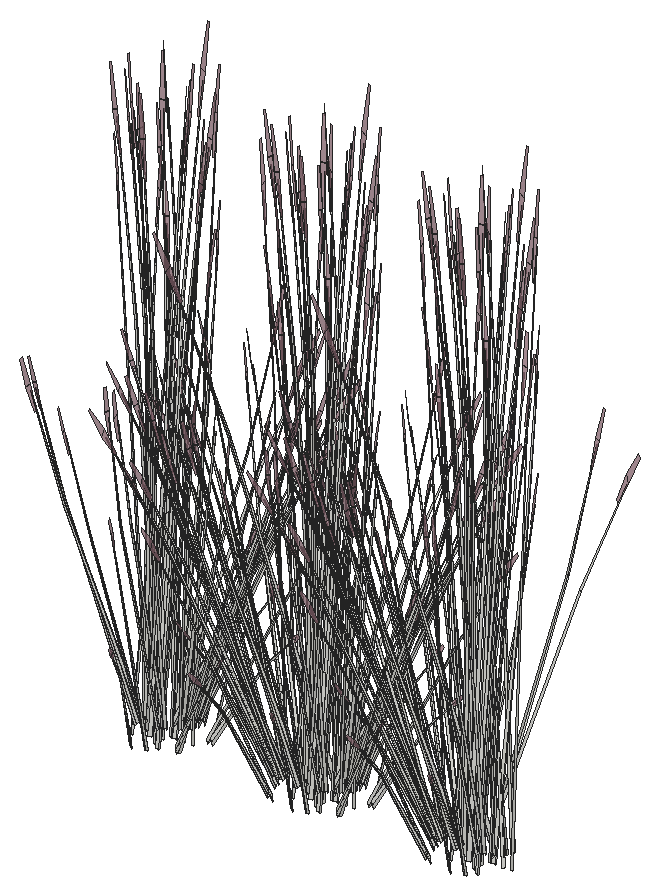
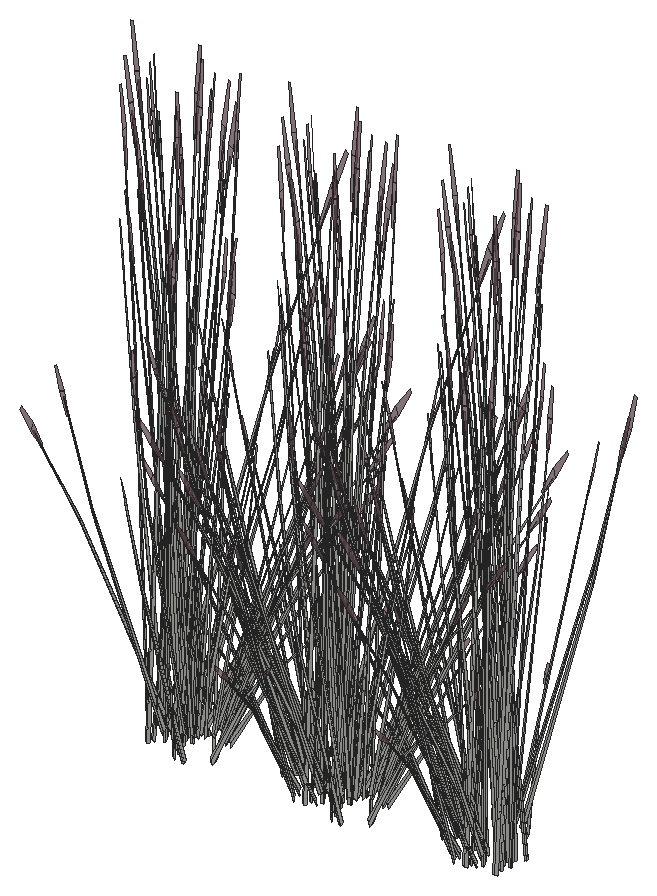
# SketchUp Ruby script. Lengths in inches.
U = 1.inch
M = Sketchup.active_model
def pt(a) = Geom::Point3d.new(a.map { |v| v * U })
def face(e, loops, mat)
  f = e.add_face(loops[0].map { |a| pt(a) })
  loops[1..].each { |l| e.add_face(l.map { |a| pt(a) }).erase! }
  f.material = f.back_material = mat if mat
  f
end
# faces: each face lists its corners as indices into pts; further lists are holes
def faces(e, pts, list, mat = nil) = list.each { |f| face(e, (f[0].is_a?(Array) ? f : [f]).map { |l| l.map { |i| pts[i] } }, mat) }
# xy, xz, yz: faces in a plane at the given z, y or x. An outline is a flat list of corners, or four numbers for a rectangle; further outlines are holes
def ring(l) = l.size == 4 ? [[l[0], l[1]], [l[2], l[1]], [l[2], l[3]], [l[0], l[3]]] : l.each_slice(2).to_a
def flat(e, list, mat, &to3) = list.each { |f| face(e, (f[0].is_a?(Array) ? f : [f]).map { |l| ring(l).map { |u, v| to3.(u, v) } }, mat) }
def xy(e, z, list, mat = nil) = flat(e, list, mat) { |x, y| [x, y, z] }
def xz(e, y, list, mat = nil) = flat(e, list, mat) { |x, z| [x, y, z] }
def yz(e, x, list, mat = nil) = flat(e, list, mat) { |y, z| [x, y, z] }
def lines(e, pts, list) = list.each { |a, b| e.add_line(pt(pts[a]), pt(pts[b])) }
# prism: a flat outline (further loops are holes) pulled along v
def prism(e, loops, v, mat = nil)
  f = face(e, loops, mat); d = Geom::Vector3d.new(v.map { |x| x * U })
  f.pushpull(f.normal.samedirection?(d) ? d.length : -d.length)
end
def box(e, o, s, mat = nil) = prism(e, [[o, [o[0] + s[0], o[1], o[2]], [o[0] + s[0], o[1] + s[1], o[2]], [o[0], o[1] + s[1], o[2]]]], [0, 0, s[2]], mat)
def at(x, y, z, deg = 0) = Geom::Transformation.translation(pt([x, y, z])) * Geom::Transformation.rotation(ORIGIN, Z_AXIS, deg.degrees)
def axes(o, x, y, z) = Geom::Transformation.new([*x, 0, *y, 0, *z, 0, *pt(o).to_a, 1])
def part(name) = M.definitions.add(name)
# library, detail: a bought-in or finely detailed component or shape, given as its bounding box
def library(name, o, s) = part(name).tap { |d| box(d.entities, o, s) }
def detail(e, o, s) = box(e.add_group.entities, o, s)
def put(e, d, t, mat = nil) = e.add_instance(d, t).tap { |i| i.material = mat if mat }
def group(e, t, mat = nil) = e.add_group.tap { |g| g.transformation = t; g.material = mat if mat }.entities
root = M.entities
M.materials.add("LightPink_Translucent").color = [144, 107, 117]
M.materials["LightPink_Translucent"].alpha = 0.75
c1 = part("blade")
p = [[2.15,0.21,22],[0,0.17,0],[0.09,0.45,0],[2.18,0.31,22],[2.29,0.31,22],[0.38,0.45,0],
  [2.48,0.24,33],[2.49,0.24,33],[2.48,0.22,33]]
faces(c1.entities,p,[[0,1,2,3],[4,5,2,3],[6,3,4,7],[8,0,3,6]])
c2 = part("seeds")
p = [[0.3,-0.1,1.38],[-0.01,-0.03,1.59],[-0.01,-0.03,0.03],[0.14,-0.07,-0.07],[0.29,-0.03,3],[0.15,0.01,3.11]]
faces(c2.entities,p,[[0,1,2,3],[1,0,4,5]],"LightPink_Translucent")
c3 = part("blade with seeds")
put(c3.entities,c1,at(0,0,0))
put(c3.entities,c2,axes([2.4,0.25,30.99],[1.5799,-0.05474,1.17369],[-0.12525,1.92788,0.29478],[-0.07173,-0.02425,1.56792]))
put(root,c3,axes([278.78,51.1875,259.68],[-0.7469,-0.15318,-0.51099],[0.25601,-0.52518,-0.3958],[-0.06849,-0.21144,0.97773]))
put(root,c3,axes([278.08,54.07,257.36],[0.96033,0.12874,0.45755],[-0.19544,0.7271,0.17955],[-0.14034,-0.07021,1.58856]))
put(root,c3,axes([277.83,53.94,257.72],[-0.36864,0.55059,0.44739],[-0.76598,-0.26498,-0.21531],[0,-0.12692,1.43643]))
put(root,c3,axes([279.05,51.29,259.98],[-0.36264,-0.49684,-0.71045],[0.74649,-0.27689,0.08574],[-0.0848,-0.24006,1.00501]))
put(root,c3,axes([277.57,55.23,257.47],[0.81646,-0.16218,0.17642],[0.20161,0.60355,0.35086],[-0.07282,-0.08794,1.60407]))
put(root,c3,axes([280,55.27,257.47],[0.21949,-0.60727,0.17642],[0.8032,0.17185,0.35086],[-0.13875,0.00296,1.60407]))
put(root,c3,axes([279.625,54.46,257.62],[0.56134,0.36712,0.1448],[-0.46823,0.41419,-0.41347],[-0.13033,0.05599,1.26744]))
put(root,c3,axes([279.61,54.19,257.72],[0.82508,-0.03772,0.44739],[0.07462,0.62614,-0.21531],[-0.14771,0.06346,1.43643]))
put(root,c3,axes([280.22,55.59,257.48],[0.7111,-0.30552,0.49651],[0.42504,0.54784,0],[-0.16196,0.06958,1.57504]))
put(root,c3,axes([279.12,50.87,259.53],[0.22906,-0.4699,-0.35414],[0.66828,0.13705,0.4572],[-0.06128,-0.18919,0.87481]))
put(root,c3,axes([278,53.4,257.36],[0.33034,0.68327,0.45755],[-0.94388,0.2376,0.17955],[0.01154,-0.12555,1.58856]))
put(root,c3,axes([281.25,53.72,257.47],[-0.59697,-0.44509,0.17642],[0.60159,-0.4317,0.35086],[-0.06593,0.0909,1.60407]))
put(root,c3,axes([278.3,53.59,257.43],[0.8561,0.29616,0.24065],[-0.41201,0.61537,0.50002],[0,-0.14185,1.60543]))
put(root,c3,axes([278.03,53.18,257.72],[-0.82508,0.03772,0.44739],[-0.07462,-0.62614,-0.21531],[0.14771,-0.06346,1.43643]))
put(root,c3,axes([277.64,52.1,257.47],[-0.21949,0.60727,0.17642],[-0.8032,-0.17185,0.35086],[0.13875,-0.00296,1.60407]))
put(root,c3,axes([280.07,52.14,257.47],[-0.81646,0.16218,0.17642],[-0.20161,-0.60355,0.35086],[0.07282,0.08794,1.60407]))
put(root,c3,axes([279.24,49.875,257.77],[0.09747,0.35631,1.1486],[-0.54071,-0.19735,0.84392],[0.05818,-0.18244,0.25299]))
put(root,c3,axes([278.74,53.02,257.36],[-0.62999,0.55453,0.45755],[-0.74845,-0.4895,0.17955],[0.15188,-0.05534,1.58856]))
put(root,c3,axes([279.81,53.43,257.72],[0.36864,-0.55059,0.44739],[0.76598,0.26498,-0.21531],[0,0.12692,1.43643]))
put(root,c3,axes([278.39,56.07,259.68],[0.7469,0.15318,-0.51099],[-0.25601,0.52518,-0.3958],[0.06849,0.21144,0.97773]))
put(root,c3,axes([279.56,53.3,257.38],[-0.96033,-0.12874,0.49198],[0.19544,-0.7271,0.19306],[0.14034,0.07021,1.70813]))
put(root,c3,axes([279.01,52.92,257.72],[-0.45644,-0.51287,0.44739],[0.69137,-0.36116,-0.21531],[0.14771,0.06346,1.43643]))
put(root,c3,axes([280.125,53.55,257.62],[0.70791,-0.1782,0.1448],[0.24791,0.50885,-0.41347],[0,0.11199,1.26744]))
put(root,c3,axes([280.39,51.59,259.68],[-0.54391,-0.41056,-0.51099],[0.57458,-0.35956,-0.3958],[0.08276,-0.2086,0.97773]))
put(root,c3,axes([280.03,50.86,257.59],[-0.21597,0.12368,1.43002],[-0.64681,-0.21647,-0.30754],[0.1199,-0.26922,0.61141]))
put(root,c3,axes([281.74,53.74,257.48],[0,-0.61104,0.49651],[0.85008,0,0],[0,0.13917,1.57504]))
put(root,c3,axes([278.82,54.98,258.875],[-0.17368,-0.19618,1.71376],[0.80256,-0.16516,0.13857],[0.18139,0.30799,0.73262]))
put(root,c3,axes([279.32,52.78,257.62],[0.14658,-0.54532,0.1448],[0.71613,0.09466,-0.41347],[0.13033,0.05599,1.26744]))
put(root,c3,axes([280.34,51.83,257.48],[-0.7111,-0.30552,0.49651],[0.42504,-0.54784,0],[0.16196,0.06958,1.57504]))
put(root,c3,axes([280.56,51.77,259.98],[0.01977,-0.56521,-0.71045],[0.83252,0.03796,0.08574],[0.08786,-0.23945,1.00501]))
put(root,c3,axes([280.9,51.43,259.53],[0.5141,-0.32171,-0.35414],[0.48666,0.36734,0.4572],[0.07405,-0.18664,0.87481]))
put(root,c3,axes([290.88,52.72,258.875],[0.31515,-0.01384,1.71376],[-0.20907,0.5998,0.13857],[-0.44912,-0.0371,0.73262]))
put(root,c3,axes([281.03,55.57,257.77],[-0.4278,-0.1757,1.1486],[0.5524,-0.17852,0.84392],[0.14899,0.15122,0.25299]))
put(root,c3,axes([279.5,55.38,257.59],[0.01341,-0.20255,1.43002],[0.64074,-0.22625,-0.30754],[0.1978,0.24243,0.61141]))
put(root,c3,axes([281.09,56.37,257.67],[-0.48723,-0.01916,1.0506],[0.32177,-0.40701,0.58006],[0.19248,0.1446,0.8241]))
put(root,c3,axes([291.01,53.77,258.875],[0.26363,-0.12925,1.71376],[0.22195,0.59723,0.13857],[-0.41388,0.13498,0.73262]))
put(root,c3,axes([290.19,54.79,257.59],[0.26405,0.05016,1.43002],[0.17019,0.51235,-0.30754],[-0.35868,0.0959,0.61141]))
put(root,c3,axes([279.62,51.49,258.875],[-0.14147,0.21002,1.71376],[-0.59349,-0.43464,0.13857],[0.26773,-0.27089,0.73262]))
put(root,c3,axes([292.53,53.15,258.34],[0.21597,-0.08839,1.77064],[0.07448,0.61717,0.13857],[-0.4678,0.08189,0.63284]))
put(root,c3,axes([280.06,55.8125,259.68],[0.74975,-0.14525,-0.51099],[0.13115,0.55007,-0.3958],[0.20138,0.15763,0.97773]))
put(root,c3,axes([291.82,52.16,259.98],[-0.75952,-0.01471,-0.71045],[0.05101,-0.61953,0.08574],[-0.32177,-0.06538,1.00501]))
put(root,c3,axes([291.21,52.31,257.59],[0.14835,0.17012,1.43002],[-0.34183,0.46242,-0.30754],[-0.351,-0.11053,0.61141]))
put(root,c3,axes([290.6,53.23,259.53],[-0.63144,-0.17046,-0.35414],[0.18417,-0.49731,0.4572],[-0.25423,0.0456,0.87481]))
put(root,c3,axes([291.48,51.75,258.875],[0.28223,0.10528,1.71376],[-0.58406,0.44165,0.13857],[-0.36402,-0.19924,0.73262]))
put(root,c3,axes([281.52,52.53,259.68],[-0.19519,-0.55794,-0.51099],[0.73919,-0.0976,-0.3958],[0.21183,-0.14986,0.97773]))
put(root,c3,axes([282.82,55.41,258.93],[-0.14542,-0.51365,-0.03492],[0.68734,-0.11809,-0.15832],[0.14353,0.03256,0.52218]))
put(root,c3,axes([291.04,53.49,259.68],[-0.20584,0.55581,-0.51099],[-0.70573,-0.19051,-0.3958],[-0.28414,0.05097,0.97773]))
put(root,c3,axes([291.57,52.28,259.68],[-0.55171,0.40476,-0.51099],[-0.48318,-0.42758,-0.3958],[-0.28031,-0.06159,0.97773]))
put(root,c3,axes([282.43,51.42,257.77],[-0.25308,0.31105,1.1486],[-0.21753,-0.4179,0.84392],[0.20902,-0.10472,0.25299]))
put(root,c3,axes([289.64,55.86,257.77],[0.31665,-0.27694,1.1486],[0.12495,0.43841,0.84392],[-0.22883,0.0785,0.25299]))
put(root,c3,axes([279.98,54.37,258.875],[-0.28223,-0.10528,1.71376],[0.58406,-0.44165,0.13857],[0.36402,0.19924,0.73262]))
put(root,c3,axes([291.37,51.9,259.53],[-0.43232,-0.38257,-0.35414],[0.49364,-0.36215,0.4572],[-0.25081,-0.0551,0.87481]))
put(root,c3,axes([291.98,54.17,258.875],[0.18977,-0.18775,1.71376],[0.47917,0.50677,0.13857],[-0.32866,0.23079,0.73262]))
put(root,c3,axes([290.83,54.67,259.53],[-0.66138,0.08733,-0.35414],[-0.17464,-0.49921,0.4572],[-0.18953,0.13408,0.87481]))
put(root,c3,axes([282.07,52.59,259.53],[0.66138,-0.08733,-0.35414],[0.17464,0.49921,0.4572],[0.18953,-0.13408,0.87481]))
put(root,c3,axes([281.54,52.76,259.98],[0.39688,-0.48213,-0.71045],[0.69548,0.34264,0.08574],[0.23697,-0.17468,1.00501]))
put(root,c3,axes([281.53,55.35,259.53],[0.43232,0.38257,-0.35414],[-0.49364,0.36215,0.4572],[0.25081,0.0551,0.87481]))
put(root,c3,axes([290.33,52.82,257.77],[0.48508,-0.04372,1.1486],[-0.3077,0.38525,0.84392],[-0.23971,-0.05779,0.25299]))
put(root,c3,axes([291.83,54.64,258.875],[0.14147,-0.21002,1.71376],[0.59349,0.43464,0.13857],[-0.26773,0.27089,0.73262]))
put(root,c3,axes([281.86,53.77,259.68],[0.20584,-0.55581,-0.51099],[0.70573,0.19051,-0.3958],[0.28414,-0.05097,0.97773]))
put(root,c3,axes([283.64,54.125,257.77],[-0.46945,0.10088,1.1486],[0.22097,-0.4169,0.84392],[0.24904,0.02853,0.25299]))
put(root,c3,axes([291.38,54.72,259.68],[0.19519,0.55794,-0.51099],[-0.73919,0.0976,-0.3958],[-0.21183,0.14986,0.97773]))
put(root,c3,axes([282.12,52.3125,257.59],[-0.27143,-0.0181,1.43002],[-0.27808,-0.48551,-0.30754],[0.33346,-0.13735,0.61141]))
put(root,c3,axes([282.3,54.02,259.53],[0.63144,0.17046,-0.35414],[-0.18417,0.49731,0.4572],[0.25423,-0.0456,0.87481]))
put(root,c3,axes([281.08,55.1,259.98],[0.75952,0.01471,-0.71045],[-0.05101,0.61953,0.08574],[0.32177,0.06538,1.00501]))
put(root,c3,axes([293.14,51.43,259.98],[-0.64788,-0.29534,-0.71045],[0.46044,-0.51755,0.08574],[-0.23473,-0.17635,1.00501]))
put(root,c3,axes([292.84,51.44,259.68],[-0.74975,0.14525,-0.51099],[-0.13115,-0.55007,-0.3958],[-0.20138,-0.15763,0.97773]))
put(root,c3,axes([280.58,53.41,258.875],[-0.31515,0.01384,1.71376],[0.20907,-0.5998,0.13857],[0.44912,0.0371,0.73262]))
put(root,c3,axes([281.73,53.97,259.98],[0.66765,-0.26986,-0.71045],[0.37208,0.55551,0.08574],[0.32259,-0.0631,1.00501]))
put(root,c3,axes([282.76,54.79,257.59],[-0.18299,-0.15028,1.43002],[0.23809,-0.49714,-0.30754],[0.37023,0.06735,0.61141]))
put(root,c3,axes([292.42,50.625,257.59],[-0.04601,0.19989,1.43002],[-0.67263,0.16733,-0.30754],[-0.15723,-0.25836,0.61141]))
put(root,c3,axes([292.64,51.14,258.875],[0.17368,0.19618,1.71376],[-0.80256,0.16516,0.13857],[-0.18139,-0.30799,0.73262]))
put(root,c3,axes([292.92,51.04,259.53],[-0.11735,-0.49217,-0.35414],[0.67083,-0.12996,0.4572],[-0.18018,-0.14104,0.87481]))
put(root,c3,axes([292,55.82,259.53],[-0.5141,0.32171,-0.35414],[-0.48666,-0.36734,0.4572],[-0.07405,0.18664,0.87481]))
put(root,c3,axes([294.69,54.77,258.33],[0.65659,0.2464,1.51261],[-0.64324,0.53082,0.59816],[-0.28812,-0.31461,1.26806]))
put(root,c3,axes([292.1875,50.3,257.77],[0.39634,0.21267,1.1486],[-0.57721,0.12784,0.84392],[-0.1235,-0.16344,0.25299]))
put(root,c3,axes([292.33,57.07,257.77],[-0.01966,-0.36332,1.1486],[0.49135,0.25914,0.84392],[-0.09663,0.17317,0.25299]))
put(root,c3,axes([293.03,55.54,257.48],[0.7111,0.30552,0.49651],[-0.42504,0.54784,0],[-0.16196,-0.06958,1.57504]))
put(root,c3,axes([294.05,54.59,257.62],[-0.14658,0.54532,0.1448],[-0.71613,-0.09466,-0.41347],[-0.13033,-0.05599,1.26744]))
put(root,c3,axes([291.625,53.63,257.48],[0,0.61104,0.49651],[-0.85008,0,0],[0,-0.13917,1.57504]))
put(root,c3,axes([292.51,55.67,260],[0.54391,0.41056,-0.5672],[-0.57458,0.35956,-0.43934],[-0.08276,0.2086,1.08528]))
put(root,c3,axes([295.71,53.59,257.84],[-0.02076,-0.57531,1.41272],[0.93937,0.14913,0.59816],[-0.22217,0.31481,1.3335]))
put(root,c3,axes([291.92,56.29,257.82],[0.69024,-0.1082,0.06507],[0.15868,0.43593,-0.86304],[-0.04376,0.22067,0.7736]))
put(root,c3,axes([294.51,51.1875,259.68],[-0.7469,-0.15318,-0.51099],[0.25601,-0.52518,-0.3958],[-0.06849,-0.21144,0.97773]))
put(root,c3,axes([293.81,54.07,257.36],[0.96033,0.12874,0.45755],[-0.19544,0.7271,0.17955],[-0.14034,-0.07021,1.58856]))
put(root,c3,axes([293.5625,53.94,257.72],[-0.36864,0.55059,0.44739],[-0.76598,-0.26498,-0.21531],[0,-0.12692,1.43643]))
put(root,c3,axes([294.78,51.29,259.98],[-0.36264,-0.49684,-0.71045],[0.74649,-0.27689,0.08574],[-0.0848,-0.24006,1.00501]))
put(root,c3,axes([293.29,55.23,257.47],[0.81646,-0.16218,0.17642],[0.20161,0.60355,0.35086],[-0.07282,-0.08794,1.60407]))
put(root,c3,axes([295.72,55.27,257.47],[0.21949,-0.60727,0.17642],[0.8032,0.17185,0.35086],[-0.13875,0.00296,1.60407]))
put(root,c3,axes([295.35,54.46,257.62],[0.56134,0.36712,0.1448],[-0.46823,0.41419,-0.41347],[-0.13033,0.05599,1.26744]))
put(root,c3,axes([295.34,54.19,257.72],[0.82508,-0.03772,0.44739],[0.07462,0.62614,-0.21531],[-0.14771,0.06346,1.43643]))
put(root,c3,axes([295.95,55.59,257.48],[0.7111,-0.30552,0.49651],[0.42504,0.54784,0],[-0.16196,0.06958,1.57504]))
put(root,c3,axes([294.85,50.87,259.53],[0.22906,-0.4699,-0.35414],[0.66828,0.13705,0.4572],[-0.06128,-0.18919,0.87481]))
put(root,c3,axes([293.73,53.4,257.36],[0.33034,0.68327,0.45755],[-0.94388,0.2376,0.17955],[0.01154,-0.12555,1.58856]))
put(root,c3,axes([296.98,53.72,257.47],[-0.59697,-0.44509,0.17642],[0.60159,-0.4317,0.35086],[-0.06593,0.0909,1.60407]))
put(root,c3,axes([294.03,53.59,257.43],[0.8561,0.29616,0.24065],[-0.41201,0.61537,0.50002],[0,-0.14185,1.60543]))
put(root,c3,axes([293.76,53.18,257.72],[-0.82508,0.03772,0.44739],[-0.07462,-0.62614,-0.21531],[0.14771,-0.06346,1.43643]))
put(root,c3,axes([293.37,52.1,257.47],[-0.21949,0.60727,0.17642],[-0.8032,-0.17185,0.35086],[0.13875,-0.00296,1.60407]))
put(root,c3,axes([295.8,52.14,257.47],[-0.81646,0.16218,0.17642],[-0.20161,-0.60355,0.35086],[0.07282,0.08794,1.60407]))
put(root,c3,axes([294.97,49.875,257.77],[0.09747,0.35631,1.1486],[-0.54071,-0.19735,0.84392],[0.05818,-0.18244,0.25299]))
put(root,c3,axes([294.46,53.02,257.36],[-0.62999,0.55453,0.45755],[-0.74845,-0.4895,0.17955],[0.15188,-0.05534,1.58856]))
put(root,c3,axes([295.53,53.43,257.72],[0.36864,-0.55059,0.44739],[0.76598,0.26498,-0.21531],[0,0.12692,1.43643]))
put(root,c3,axes([294.12,56.07,259.68],[0.7469,0.15318,-0.51099],[-0.25601,0.52518,-0.3958],[0.06849,0.21144,0.97773]))
put(root,c3,axes([295.29,53.3,257.38],[-0.96033,-0.12874,0.49198],[0.19544,-0.7271,0.19306],[0.14034,0.07021,1.70813]))
put(root,c3,axes([294.74,52.92,257.72],[-0.45644,-0.51287,0.44739],[0.69137,-0.36116,-0.21531],[0.14771,0.06346,1.43643]))
put(root,c3,axes([295.85,53.55,257.62],[0.70791,-0.1782,0.1448],[0.24791,0.50885,-0.41347],[0,0.11199,1.26744]))
put(root,c3,axes([296.12,51.59,259.68],[-0.54391,-0.41056,-0.51099],[0.57458,-0.35956,-0.3958],[0.08276,-0.2086,0.97773]))
put(root,c3,axes([295.76,50.86,257.59],[-0.21597,0.12368,1.43002],[-0.64681,-0.21647,-0.30754],[0.1199,-0.26922,0.61141]))
put(root,c3,axes([297.47,53.74,257.48],[0,-0.61104,0.49651],[0.85008,0,0],[0,0.13917,1.57504]))
put(root,c3,axes([294.55,54.98,258.875],[-0.17368,-0.19618,1.71376],[0.80256,-0.16516,0.13857],[0.18139,0.30799,0.73262]))
put(root,c3,axes([295.05,52.78,257.62],[0.14658,-0.54532,0.1448],[0.71613,0.09466,-0.41347],[0.13033,0.05599,1.26744]))
put(root,c3,axes([296.07,51.83,257.48],[-0.7111,-0.30552,0.49651],[0.42504,-0.54784,0],[0.16196,0.06958,1.57504]))
put(root,c3,axes([296.29,51.77,259.98],[0.01977,-0.56521,-0.71045],[0.83252,0.03796,0.08574],[0.08786,-0.23945,1.00501]))
put(root,c3,axes([306.33,52.72,258.875],[0.31515,-0.01384,1.71376],[-0.20907,0.5998,0.13857],[-0.44912,-0.0371,0.73262]))
put(root,c3,axes([296.63,51.43,259.53],[0.5141,-0.32171,-0.35414],[0.48666,0.36734,0.4572],[0.07405,-0.18664,0.87481]))
put(root,c3,axes([296.75,55.57,257.77],[-0.4278,-0.1757,1.1486],[0.5524,-0.17852,0.84392],[0.14899,0.15122,0.25299]))
put(root,c3,axes([295.23,55.38,257.59],[0.01341,-0.20255,1.43002],[0.64074,-0.22625,-0.30754],[0.1978,0.24243,0.61141]))
put(root,c3,axes([306.46,53.77,258.875],[0.26363,-0.12925,1.71376],[0.22195,0.59723,0.13857],[-0.41388,0.13498,0.73262]))
put(root,c3,axes([305.64,54.79,257.59],[0.26405,0.05016,1.43002],[0.17019,0.51235,-0.30754],[-0.35868,0.0959,0.61141]))
put(root,c3,axes([296.82,56.37,257.67],[-0.48723,-0.01916,1.0506],[0.32177,-0.40701,0.58006],[0.19248,0.1446,0.8241]))
put(root,c3,axes([307.97,53.15,258.34],[0.21597,-0.08839,1.77064],[0.07448,0.61717,0.13857],[-0.4678,0.08189,0.63284]))
put(root,c3,axes([295.35,51.49,258.875],[-0.14147,0.21002,1.71376],[-0.59349,-0.43464,0.13857],[0.26773,-0.27089,0.73262]))
put(root,c3,axes([307.27,52.16,259.98],[-0.75952,-0.01471,-0.71045],[0.05101,-0.61953,0.08574],[-0.32177,-0.06538,1.00501]))
put(root,c3,axes([306.66,52.31,257.59],[0.14835,0.17012,1.43002],[-0.34183,0.46242,-0.30754],[-0.351,-0.11053,0.61141]))
put(root,c3,axes([295.79,55.8125,259.68],[0.74975,-0.14525,-0.51099],[0.13115,0.55007,-0.3958],[0.20138,0.15763,0.97773]))
put(root,c3,axes([306.05,53.23,259.53],[-0.63144,-0.17046,-0.35414],[0.18417,-0.49731,0.4572],[-0.25423,0.0456,0.87481]))
put(root,c3,axes([306.92,51.75,258.875],[0.28223,0.10528,1.71376],[-0.58406,0.44165,0.13857],[-0.36402,-0.19924,0.73262]))
put(root,c3,axes([306.48,53.49,259.68],[-0.20584,0.55581,-0.51099],[-0.70573,-0.19051,-0.3958],[-0.28414,0.05097,0.97773]))
put(root,c3,axes([297.25,52.53,259.68],[-0.19519,-0.55794,-0.51099],[0.73919,-0.0976,-0.3958],[0.21183,-0.14986,0.97773]))
put(root,c3,axes([307.02,52.28,259.68],[-0.55171,0.40476,-0.51099],[-0.48318,-0.42758,-0.3958],[-0.28031,-0.06159,0.97773]))
put(root,c3,axes([298.55,55.41,258.93],[-0.14542,-0.51365,-0.03492],[0.68734,-0.11809,-0.15832],[0.14353,0.03256,0.52218]))
put(root,c3,axes([305.09,55.86,257.77],[0.31665,-0.27694,1.1486],[0.12495,0.43841,0.84392],[-0.22883,0.0785,0.25299]))
put(root,c3,axes([298.16,51.42,257.77],[-0.25308,0.31105,1.1486],[-0.21753,-0.4179,0.84392],[0.20902,-0.10472,0.25299]))
put(root,c3,axes([306.81,51.9,259.53],[-0.43232,-0.38257,-0.35414],[0.49364,-0.36215,0.4572],[-0.25081,-0.0551,0.87481]))
put(root,c3,axes([307.42,54.17,258.875],[0.18977,-0.18775,1.71376],[0.47917,0.50677,0.13857],[-0.32866,0.23079,0.73262]))
put(root,c3,axes([306.28,54.67,259.53],[-0.66138,0.08733,-0.35414],[-0.17464,-0.49921,0.4572],[-0.18953,0.13408,0.87481]))
put(root,c3,axes([295.71,54.37,258.875],[-0.28223,-0.10528,1.71376],[0.58406,-0.44165,0.13857],[0.36402,0.19924,0.73262]))
put(root,c3,axes([305.78,52.82,257.77],[0.48508,-0.04372,1.1486],[-0.3077,0.38525,0.84392],[-0.23971,-0.05779,0.25299]))
put(root,c3,axes([297.79,52.59,259.53],[0.66138,-0.08733,-0.35414],[0.17464,0.49921,0.4572],[0.18953,-0.13408,0.87481]))
put(root,c3,axes([297.27,52.76,259.98],[0.39688,-0.48213,-0.71045],[0.69548,0.34264,0.08574],[0.23697,-0.17468,1.00501]))
put(root,c3,axes([297.26,55.35,259.53],[0.43232,0.38257,-0.35414],[-0.49364,0.36215,0.4572],[0.25081,0.0551,0.87481]))
put(root,c3,axes([307.28,54.64,258.875],[0.14147,-0.21002,1.71376],[0.59349,0.43464,0.13857],[-0.26773,0.27089,0.73262]))
put(root,c3,axes([306.83,54.72,259.68],[0.19519,0.55794,-0.51099],[-0.73919,0.0976,-0.3958],[-0.21183,0.14986,0.97773]))
put(root,c3,axes([297.59,53.77,259.68],[0.20584,-0.55581,-0.51099],[0.70573,0.19051,-0.3958],[0.28414,-0.05097,0.97773]))
put(root,c3,axes([299.36,54.125,257.77],[-0.46945,0.10088,1.1486],[0.22097,-0.4169,0.84392],[0.24904,0.02853,0.25299]))
put(root,c3,axes([297.84,52.3125,257.59],[-0.27143,-0.0181,1.43002],[-0.27808,-0.48551,-0.30754],[0.33346,-0.13735,0.61141]))
put(root,c3,axes([298.03,54.02,259.53],[0.63144,0.17046,-0.35414],[-0.18417,0.49731,0.4572],[0.25423,-0.0456,0.87481]))
put(root,c3,axes([308.59,51.43,259.98],[-0.64788,-0.29534,-0.71045],[0.46044,-0.51755,0.08574],[-0.23473,-0.17635,1.00501]))
put(root,c3,axes([308.29,51.44,259.68],[-0.74975,0.14525,-0.51099],[-0.13115,-0.55007,-0.3958],[-0.20138,-0.15763,0.97773]))
put(root,c3,axes([296.81,55.1,259.98],[0.75952,0.01471,-0.71045],[-0.05101,0.61953,0.08574],[0.32177,0.06538,1.00501]))
put(root,c3,axes([296.3,53.41,258.875],[-0.31515,0.01384,1.71376],[0.20907,-0.5998,0.13857],[0.44912,0.0371,0.73262]))
put(root,c3,axes([297.46,53.97,259.98],[0.66765,-0.26986,-0.71045],[0.37208,0.55551,0.08574],[0.32259,-0.0631,1.00501]))
put(root,c3,axes([307.87,50.625,257.59],[-0.04601,0.19989,1.43002],[-0.67263,0.16733,-0.30754],[-0.15723,-0.25836,0.61141]))
put(root,c3,axes([308.09,51.14,258.875],[0.17368,0.19618,1.71376],[-0.80256,0.16516,0.13857],[-0.18139,-0.30799,0.73262]))
put(root,c3,axes([298.48,54.79,257.59],[-0.18299,-0.15028,1.43002],[0.23809,-0.49714,-0.30754],[0.37023,0.06735,0.61141]))
put(root,c3,axes([308.37,51.04,259.53],[-0.11735,-0.49217,-0.35414],[0.67083,-0.12996,0.4572],[-0.18018,-0.14104,0.87481]))
put(root,c3,axes([307.45,55.82,259.53],[-0.5141,0.32171,-0.35414],[-0.48666,-0.36734,0.4572],[-0.07405,0.18664,0.87481]))
put(root,c3,axes([310.14,54.77,258.33],[0.65659,0.2464,1.51261],[-0.64324,0.53082,0.59816],[-0.28812,-0.31461,1.26806]))
put(root,c3,axes([307.64,50.3,257.77],[0.39634,0.21267,1.1486],[-0.57721,0.12784,0.84392],[-0.1235,-0.16344,0.25299]))
put(root,c3,axes([307.77,57.07,257.77],[-0.01966,-0.36332,1.1486],[0.49135,0.25914,0.84392],[-0.09663,0.17317,0.25299]))
put(root,c3,axes([308.48,55.54,257.48],[0.7111,0.30552,0.49651],[-0.42504,0.54784,0],[-0.16196,-0.06958,1.57504]))
put(root,c3,axes([309.49,54.59,257.62],[-0.14658,0.54532,0.1448],[-0.71613,-0.09466,-0.41347],[-0.13033,-0.05599,1.26744]))
put(root,c3,axes([307.07,53.63,257.48],[0,0.61104,0.49651],[-0.85008,0,0],[0,-0.13917,1.57504]))
put(root,c3,axes([307.96,55.67,260],[0.54391,0.41056,-0.5672],[-0.57458,0.35956,-0.43934],[-0.08276,0.2086,1.08528]))
put(root,c3,axes([311.16,53.59,257.84],[-0.02076,-0.57531,1.41272],[0.93937,0.14913,0.59816],[-0.22217,0.31481,1.3335]))
put(root,c3,axes([307.37,56.29,257.82],[0.69024,-0.1082,0.06507],[0.15868,0.43593,-0.86304],[-0.04376,0.22067,0.7736]))
put(root,c3,axes([309.95,51.1875,259.68],[-0.7469,-0.15318,-0.51099],[0.25601,-0.52518,-0.3958],[-0.06849,-0.21144,0.97773]))
put(root,c3,axes([309.26,54.07,257.36],[0.96033,0.12874,0.45755],[-0.19544,0.7271,0.17955],[-0.14034,-0.07021,1.58856]))
put(root,c3,axes([309.01,53.94,257.72],[-0.36864,0.55059,0.44739],[-0.76598,-0.26498,-0.21531],[0,-0.12692,1.43643]))
put(root,c3,axes([310.23,51.29,259.98],[-0.36264,-0.49684,-0.71045],[0.74649,-0.27689,0.08574],[-0.0848,-0.24006,1.00501]))
put(root,c3,axes([308.74,55.23,257.47],[0.81646,-0.16218,0.17642],[0.20161,0.60355,0.35086],[-0.07282,-0.08794,1.60407]))
put(root,c3,axes([311.17,55.27,257.47],[0.21949,-0.60727,0.17642],[0.8032,0.17185,0.35086],[-0.13875,0.00296,1.60407]))
put(root,c3,axes([310.8,54.46,257.62],[0.56134,0.36712,0.1448],[-0.46823,0.41419,-0.41347],[-0.13033,0.05599,1.26744]))
put(root,c3,axes([310.79,54.19,257.72],[0.82508,-0.03772,0.44739],[0.07462,0.62614,-0.21531],[-0.14771,0.06346,1.43643]))
put(root,c3,axes([311.4,55.59,257.48],[0.7111,-0.30552,0.49651],[0.42504,0.54784,0],[-0.16196,0.06958,1.57504]))
put(root,c3,axes([310.29,50.87,259.53],[0.22906,-0.4699,-0.35414],[0.66828,0.13705,0.4572],[-0.06128,-0.18919,0.87481]))
put(root,c3,axes([309.18,53.4,257.36],[0.33034,0.68327,0.45755],[-0.94388,0.2376,0.17955],[0.01154,-0.12555,1.58856]))
put(root,c3,axes([312.43,53.72,257.47],[-0.59697,-0.44509,0.17642],[0.60159,-0.4317,0.35086],[-0.06593,0.0909,1.60407]))
put(root,c3,axes([309.48,53.59,257.43],[0.8561,0.29616,0.24065],[-0.41201,0.61537,0.50002],[0,-0.14185,1.60543]))
put(root,c3,axes([309.2,53.18,257.72],[-0.82508,0.03772,0.44739],[-0.07462,-0.62614,-0.21531],[0.14771,-0.06346,1.43643]))
put(root,c3,axes([308.82,52.1,257.47],[-0.21949,0.60727,0.17642],[-0.8032,-0.17185,0.35086],[0.13875,-0.00296,1.60407]))
put(root,c3,axes([311.25,52.14,257.47],[-0.81646,0.16218,0.17642],[-0.20161,-0.60355,0.35086],[0.07282,0.08794,1.60407]))
put(root,c3,axes([310.42,49.875,257.77],[0.09747,0.35631,1.1486],[-0.54071,-0.19735,0.84392],[0.05818,-0.18244,0.25299]))
put(root,c3,axes([309.91,53.02,257.36],[-0.62999,0.55453,0.45755],[-0.74845,-0.4895,0.17955],[0.15188,-0.05534,1.58856]))
put(root,c3,axes([310.98,53.43,257.72],[0.36864,-0.55059,0.44739],[0.76598,0.26498,-0.21531],[0,0.12692,1.43643]))
put(root,c3,axes([309.57,56.07,259.68],[0.7469,0.15318,-0.51099],[-0.25601,0.52518,-0.3958],[0.06849,0.21144,0.97773]))
put(root,c3,axes([310.73,53.3,257.38],[-0.96033,-0.12874,0.49198],[0.19544,-0.7271,0.19306],[0.14034,0.07021,1.70813]))
put(root,c3,axes([310.19,52.92,257.72],[-0.45644,-0.51287,0.44739],[0.69137,-0.36116,-0.21531],[0.14771,0.06346,1.43643]))
put(root,c3,axes([311.3,53.55,257.62],[0.70791,-0.1782,0.1448],[0.24791,0.50885,-0.41347],[0,0.11199,1.26744]))
put(root,c3,axes([311.57,51.59,259.68],[-0.54391,-0.41056,-0.51099],[0.57458,-0.35956,-0.3958],[0.08276,-0.2086,0.97773]))
put(root,c3,axes([311.21,50.86,257.59],[-0.21597,0.12368,1.43002],[-0.64681,-0.21647,-0.30754],[0.1199,-0.26922,0.61141]))
put(root,c3,axes([312.92,53.74,257.48],[0,-0.61104,0.49651],[0.85008,0,0],[0,0.13917,1.57504]))
put(root,c3,axes([309.99,54.98,258.875],[-0.17368,-0.19618,1.71376],[0.80256,-0.16516,0.13857],[0.18139,0.30799,0.73262]))
put(root,c3,axes([310.5,52.78,257.62],[0.14658,-0.54532,0.1448],[0.71613,0.09466,-0.41347],[0.13033,0.05599,1.26744]))
put(root,c3,axes([311.52,51.83,257.48],[-0.7111,-0.30552,0.49651],[0.42504,-0.54784,0],[0.16196,0.06958,1.57504]))
put(root,c3,axes([311.74,51.77,259.98],[0.01977,-0.56521,-0.71045],[0.83252,0.03796,0.08574],[0.08786,-0.23945,1.00501]))
put(root,c3,axes([312.08,51.43,259.53],[0.5141,-0.32171,-0.35414],[0.48666,0.36734,0.4572],[0.07405,-0.18664,0.87481]))
